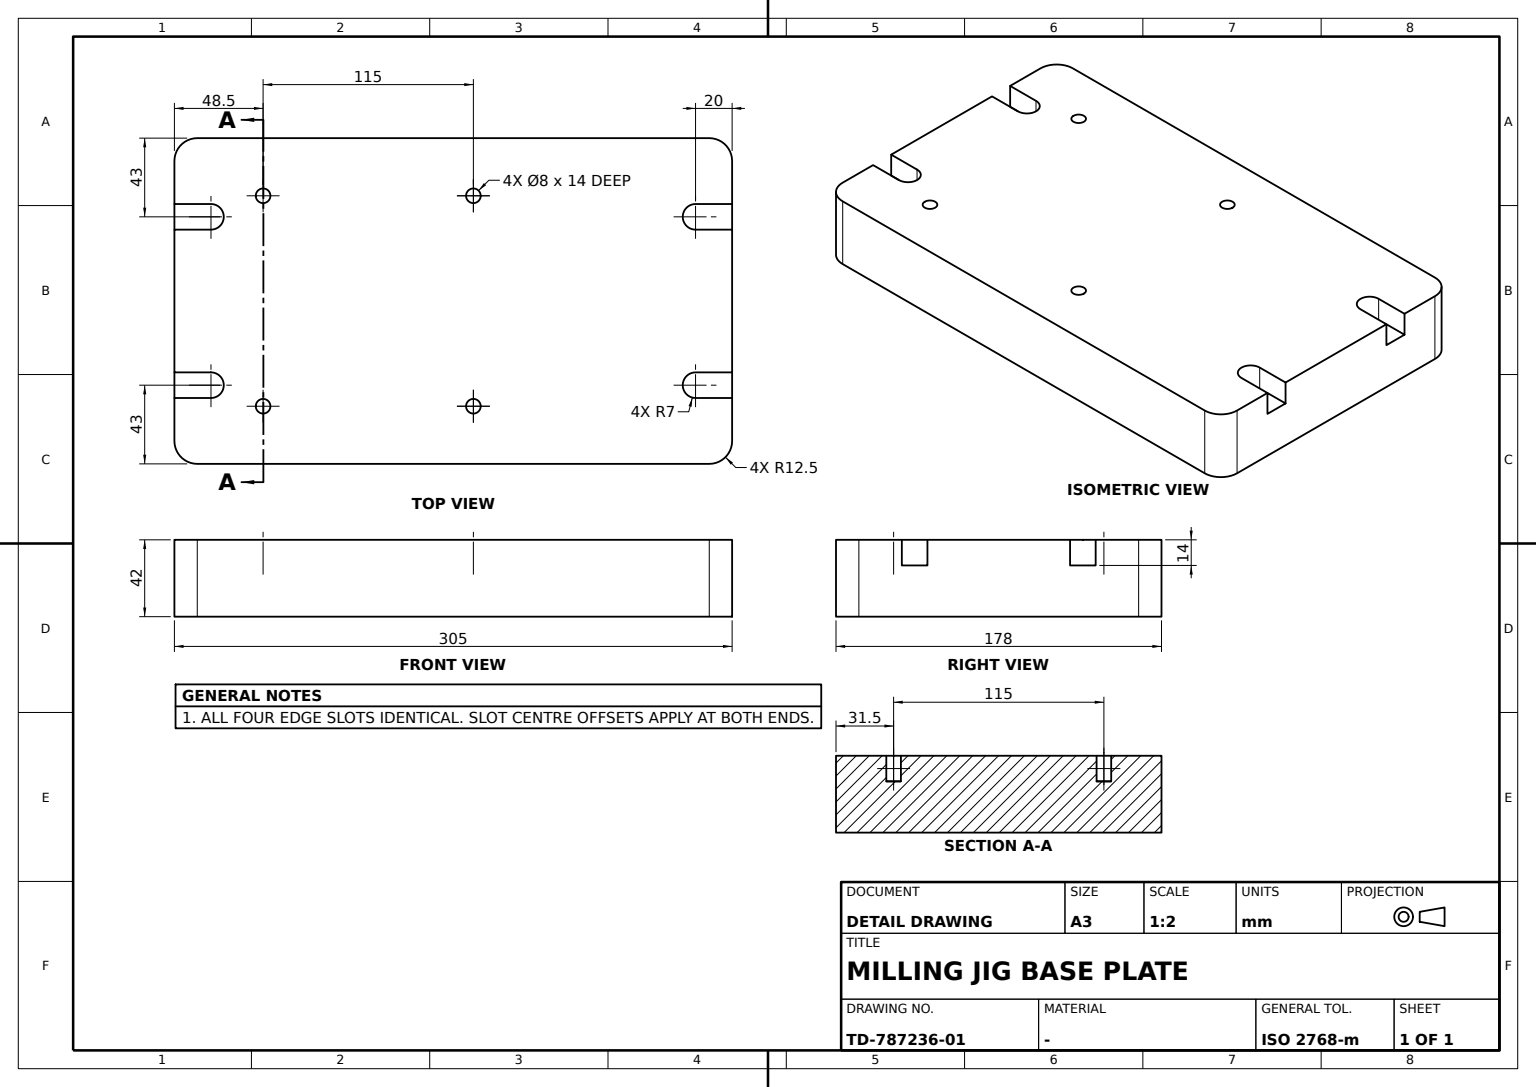
ISO-10303-21;
HEADER;
FILE_DESCRIPTION((''),'2;1');
FILE_NAME('','',(''),(''),'','','');
FILE_SCHEMA(('AUTOMOTIVE_DESIGN'));
ENDSEC;
DATA;
#1=APPLICATION_CONTEXT('');
#2=PRODUCT_CONTEXT('',#1,'mechanical');
#3=PRODUCT('','','',(#2));
#4=PRODUCT_DEFINITION_FORMATION('','',#3);
#5=PRODUCT_DEFINITION_CONTEXT('',#1,'design');
#6=PRODUCT_DEFINITION('','',#4,#5);
#7=PRODUCT_DEFINITION_SHAPE('','',#6);
#8=(LENGTH_UNIT()NAMED_UNIT(*)SI_UNIT(.MILLI.,.METRE.));
#9=(NAMED_UNIT(*)PLANE_ANGLE_UNIT()SI_UNIT($,.RADIAN.));
#10=(NAMED_UNIT(*)SI_UNIT($,.STERADIAN.)SOLID_ANGLE_UNIT());
#11=UNCERTAINTY_MEASURE_WITH_UNIT(LENGTH_MEASURE(1.E-05),#8,'distance_accuracy_value','');
#12=(GEOMETRIC_REPRESENTATION_CONTEXT(3)GLOBAL_UNCERTAINTY_ASSIGNED_CONTEXT((#11))GLOBAL_UNIT_ASSIGNED_CONTEXT((#8,#9,#10))REPRESENTATION_CONTEXT('',''));
#13=CARTESIAN_POINT('',(89.,140.,28.));
#14=VERTEX_POINT('',#13);
#15=CARTESIAN_POINT('',(89.,140.,-14.));
#16=VERTEX_POINT('',#15);
#17=CARTESIAN_POINT('',(89.,140.,7.));
#18=DIRECTION('',(0.,0.,-1.));
#19=VECTOR('',#18,1000.);
#20=LINE('',#17,#19);
#21=EDGE_CURVE('',#14,#16,#20,.T.);
#22=ORIENTED_EDGE('',*,*,#21,.F.);
#23=CARTESIAN_POINT('',(89.,-140.,28.));
#24=VERTEX_POINT('',#23);
#25=CARTESIAN_POINT('',(89.,0.,28.));
#26=DIRECTION('',(0.,1.,0.));
#27=VECTOR('',#26,1000.);
#28=LINE('',#25,#27);
#29=EDGE_CURVE('',#24,#14,#28,.T.);
#30=ORIENTED_EDGE('',*,*,#29,.F.);
#31=CARTESIAN_POINT('',(89.,-140.,-14.));
#32=VERTEX_POINT('',#31);
#33=CARTESIAN_POINT('',(89.,-140.,7.));
#34=LINE('',#33,#19);
#35=EDGE_CURVE('',#24,#32,#34,.T.);
#36=ORIENTED_EDGE('',*,*,#35,.T.);
#37=CARTESIAN_POINT('',(89.,0.,-14.));
#38=LINE('',#37,#27);
#39=EDGE_CURVE('',#32,#16,#38,.T.);
#40=ORIENTED_EDGE('',*,*,#39,.T.);
#41=EDGE_LOOP('',(#22,#30,#36,#40));
#42=FACE_OUTER_BOUND('',#41,.T.);
#43=CARTESIAN_POINT('',(89.,140.,0.));
#44=DIRECTION('',(1.,0.,0.));
#45=DIRECTION('',(0.,-1.,0.));
#46=AXIS2_PLACEMENT_3D('',#43,#44,#45);
#47=PLANE('',#46);
#48=ADVANCED_FACE('',(#42),#47,.T.);
#49=CARTESIAN_POINT('',(-89.,-140.,28.));
#50=VERTEX_POINT('',#49);
#51=CARTESIAN_POINT('',(-89.,-140.,-14.));
#52=VERTEX_POINT('',#51);
#53=CARTESIAN_POINT('',(-89.,-140.,7.));
#54=LINE('',#53,#19);
#55=EDGE_CURVE('',#50,#52,#54,.T.);
#56=ORIENTED_EDGE('',*,*,#55,.T.);
#57=CARTESIAN_POINT('',(-76.5,-152.5,-14.));
#58=VERTEX_POINT('',#57);
#59=CARTESIAN_POINT('',(-76.5,-140.,-14.));
#60=DIRECTION('',(0.,0.,1.));
#61=AXIS2_PLACEMENT_3D('',#59,#60,#26);
#62=CIRCLE('',#61,12.5);
#63=EDGE_CURVE('',#52,#58,#62,.T.);
#64=ORIENTED_EDGE('',*,*,#63,.T.);
#65=CARTESIAN_POINT('',(-76.5,-152.5,28.));
#66=VERTEX_POINT('',#65);
#67=CARTESIAN_POINT('',(-76.5,-152.5,7.));
#68=LINE('',#67,#19);
#69=EDGE_CURVE('',#66,#58,#68,.T.);
#70=ORIENTED_EDGE('',*,*,#69,.F.);
#71=CARTESIAN_POINT('',(-76.5,-140.,28.));
#72=AXIS2_PLACEMENT_3D('',#71,#60,#26);
#73=CIRCLE('',#72,12.5);
#74=EDGE_CURVE('',#50,#66,#73,.T.);
#75=ORIENTED_EDGE('',*,*,#74,.F.);
#76=EDGE_LOOP('',(#56,#64,#70,#75));
#77=FACE_OUTER_BOUND('',#76,.T.);
#78=CARTESIAN_POINT('',(-76.5,-140.,0.));
#79=AXIS2_PLACEMENT_3D('',#78,#18,#26);
#80=CYLINDRICAL_SURFACE('',#79,12.5);
#81=ADVANCED_FACE('',(#77),#80,.T.);
#82=CARTESIAN_POINT('',(-53.,132.5,0.));
#83=VERTEX_POINT('',#82);
#84=CARTESIAN_POINT('',(-53.,132.5,-14.));
#85=VERTEX_POINT('',#84);
#86=CARTESIAN_POINT('',(-53.,132.5,15.5));
#87=LINE('',#86,#19);
#88=EDGE_CURVE('',#83,#85,#87,.T.);
#89=ORIENTED_EDGE('',*,*,#88,.T.);
#90=CARTESIAN_POINT('',(-53.,152.5,-14.));
#91=VERTEX_POINT('',#90);
#92=CARTESIAN_POINT('',(-53.,142.5,-14.));
#93=VECTOR('',#45,1000.);
#94=LINE('',#92,#93);
#95=EDGE_CURVE('',#91,#85,#94,.T.);
#96=ORIENTED_EDGE('',*,*,#95,.F.);
#97=CARTESIAN_POINT('',(-53.,152.5,0.));
#98=VERTEX_POINT('',#97);
#99=CARTESIAN_POINT('',(-53.,152.5,-7.));
#100=LINE('',#99,#19);
#101=EDGE_CURVE('',#98,#91,#100,.T.);
#102=ORIENTED_EDGE('',*,*,#101,.F.);
#103=CARTESIAN_POINT('',(-53.,142.5,0.));
#104=LINE('',#103,#93);
#105=EDGE_CURVE('',#98,#83,#104,.T.);
#106=ORIENTED_EDGE('',*,*,#105,.T.);
#107=EDGE_LOOP('',(#89,#96,#102,#106));
#108=FACE_OUTER_BOUND('',#107,.T.);
#109=CARTESIAN_POINT('',(-53.,-132.5,14.));
#110=AXIS2_PLACEMENT_3D('',#109,#44,#45);
#111=PLANE('',#110);
#112=ADVANCED_FACE('',(#108),#111,.T.);
#113=CARTESIAN_POINT('',(76.5,-152.5,28.));
#114=VERTEX_POINT('',#113);
#115=CARTESIAN_POINT('',(0.,-152.5,28.));
#116=VECTOR('',#44,1000.);
#117=LINE('',#115,#116);
#118=EDGE_CURVE('',#66,#114,#117,.T.);
#119=ORIENTED_EDGE('',*,*,#118,.T.);
#120=CARTESIAN_POINT('',(76.5,-140.,28.));
#121=AXIS2_PLACEMENT_3D('',#120,#60,#26);
#122=CIRCLE('',#121,12.5);
#123=EDGE_CURVE('',#114,#24,#122,.T.);
#124=ORIENTED_EDGE('',*,*,#123,.T.);
#125=ORIENTED_EDGE('',*,*,#29,.T.);
#126=CARTESIAN_POINT('',(76.5,152.5,28.));
#127=VERTEX_POINT('',#126);
#128=CARTESIAN_POINT('',(76.5,140.,28.));
#129=AXIS2_PLACEMENT_3D('',#128,#60,#26);
#130=CIRCLE('',#129,12.5);
#131=EDGE_CURVE('',#14,#127,#130,.T.);
#132=ORIENTED_EDGE('',*,*,#131,.T.);
#133=CARTESIAN_POINT('',(-76.5,152.5,28.));
#134=VERTEX_POINT('',#133);
#135=CARTESIAN_POINT('',(0.,152.5,28.));
#136=DIRECTION('',(-1.,0.,0.));
#137=VECTOR('',#136,1000.);
#138=LINE('',#135,#137);
#139=EDGE_CURVE('',#127,#134,#138,.T.);
#140=ORIENTED_EDGE('',*,*,#139,.T.);
#141=CARTESIAN_POINT('',(-89.,140.,28.));
#142=VERTEX_POINT('',#141);
#143=CARTESIAN_POINT('',(-76.5,140.,28.));
#144=AXIS2_PLACEMENT_3D('',#143,#60,#26);
#145=CIRCLE('',#144,12.5);
#146=EDGE_CURVE('',#134,#142,#145,.T.);
#147=ORIENTED_EDGE('',*,*,#146,.T.);
#148=CARTESIAN_POINT('',(-89.,0.,28.));
#149=LINE('',#148,#93);
#150=EDGE_CURVE('',#142,#50,#149,.T.);
#151=ORIENTED_EDGE('',*,*,#150,.T.);
#152=ORIENTED_EDGE('',*,*,#74,.T.);
#153=EDGE_LOOP('',(#119,#124,#125,#132,#140,#147,#151,#152));
#154=FACE_OUTER_BOUND('',#153,.T.);
#155=CARTESIAN_POINT('',(0.,0.,28.));
#156=AXIS2_PLACEMENT_3D('',#155,#60,#26);
#157=PLANE('',#156);
#158=ADVANCED_FACE('',(#154),#157,.T.);
#159=CARTESIAN_POINT('',(-57.5,-108.,0.));
#160=VERTEX_POINT('',#159);
#161=CARTESIAN_POINT('',(-57.5,-100.,0.));
#162=VERTEX_POINT('',#161);
#163=CARTESIAN_POINT('',(-57.5,-104.,0.));
#164=AXIS2_PLACEMENT_3D('',#163,#60,#26);
#165=CIRCLE('',#164,4.);
#166=EDGE_CURVE('',#160,#162,#165,.T.);
#167=ORIENTED_EDGE('',*,*,#166,.T.);
#168=CARTESIAN_POINT('',(-57.5,-100.,-14.));
#169=VERTEX_POINT('',#168);
#170=CARTESIAN_POINT('',(-57.5,-100.,0.84));
#171=LINE('',#170,#19);
#172=EDGE_CURVE('',#162,#169,#171,.T.);
#173=ORIENTED_EDGE('',*,*,#172,.T.);
#174=CARTESIAN_POINT('',(-57.5,-108.,-14.));
#175=VERTEX_POINT('',#174);
#176=CARTESIAN_POINT('',(-57.5,-104.,-14.));
#177=AXIS2_PLACEMENT_3D('',#176,#60,#26);
#178=CIRCLE('',#177,4.);
#179=EDGE_CURVE('',#175,#169,#178,.T.);
#180=ORIENTED_EDGE('',*,*,#179,.F.);
#181=CARTESIAN_POINT('',(-57.5,-108.,0.84));
#182=LINE('',#181,#19);
#183=EDGE_CURVE('',#160,#175,#182,.T.);
#184=ORIENTED_EDGE('',*,*,#183,.F.);
#185=EDGE_LOOP('',(#167,#173,#180,#184));
#186=FACE_OUTER_BOUND('',#185,.T.);
#187=CARTESIAN_POINT('',(-57.5,-104.,0.84));
#188=AXIS2_PLACEMENT_3D('',#187,#18,#26);
#189=CYLINDRICAL_SURFACE('',#188,4.);
#190=ADVANCED_FACE('',(#186),#189,.F.);
#191=CARTESIAN_POINT('',(-39.,132.5,0.));
#192=VERTEX_POINT('',#191);
#193=CARTESIAN_POINT('',(-46.,132.5,0.));
#194=AXIS2_PLACEMENT_3D('',#193,#60,#26);
#195=CIRCLE('',#194,7.);
#196=EDGE_CURVE('',#83,#192,#195,.T.);
#197=ORIENTED_EDGE('',*,*,#196,.T.);
#198=CARTESIAN_POINT('',(-39.,132.5,-14.));
#199=VERTEX_POINT('',#198);
#200=CARTESIAN_POINT('',(-39.,132.5,15.5));
#201=LINE('',#200,#19);
#202=EDGE_CURVE('',#192,#199,#201,.T.);
#203=ORIENTED_EDGE('',*,*,#202,.T.);
#204=CARTESIAN_POINT('',(-46.,132.5,-14.));
#205=AXIS2_PLACEMENT_3D('',#204,#60,#26);
#206=CIRCLE('',#205,7.);
#207=EDGE_CURVE('',#85,#199,#206,.T.);
#208=ORIENTED_EDGE('',*,*,#207,.F.);
#209=ORIENTED_EDGE('',*,*,#88,.F.);
#210=EDGE_LOOP('',(#197,#203,#208,#209));
#211=FACE_OUTER_BOUND('',#210,.T.);
#212=CARTESIAN_POINT('',(-46.,132.5,15.5));
#213=AXIS2_PLACEMENT_3D('',#212,#18,#26);
#214=CYLINDRICAL_SURFACE('',#213,7.);
#215=ADVANCED_FACE('',(#211),#214,.F.);
#216=CARTESIAN_POINT('',(-57.5,15.,0.));
#217=VERTEX_POINT('',#216);
#218=CARTESIAN_POINT('',(-57.5,15.,-14.));
#219=VERTEX_POINT('',#218);
#220=CARTESIAN_POINT('',(-57.5,15.,0.84));
#221=LINE('',#220,#19);
#222=EDGE_CURVE('',#217,#219,#221,.T.);
#223=ORIENTED_EDGE('',*,*,#222,.F.);
#224=CARTESIAN_POINT('',(-57.5,7.,0.));
#225=VERTEX_POINT('',#224);
#226=CARTESIAN_POINT('',(-57.5,11.,0.));
#227=AXIS2_PLACEMENT_3D('',#226,#60,#26);
#228=CIRCLE('',#227,4.);
#229=EDGE_CURVE('',#217,#225,#228,.T.);
#230=ORIENTED_EDGE('',*,*,#229,.T.);
#231=CARTESIAN_POINT('',(-57.5,7.,-14.));
#232=VERTEX_POINT('',#231);
#233=CARTESIAN_POINT('',(-57.5,7.,0.84));
#234=LINE('',#233,#19);
#235=EDGE_CURVE('',#225,#232,#234,.T.);
#236=ORIENTED_EDGE('',*,*,#235,.T.);
#237=CARTESIAN_POINT('',(-57.5,11.,-14.));
#238=AXIS2_PLACEMENT_3D('',#237,#60,#26);
#239=CIRCLE('',#238,4.);
#240=EDGE_CURVE('',#219,#232,#239,.T.);
#241=ORIENTED_EDGE('',*,*,#240,.F.);
#242=EDGE_LOOP('',(#223,#230,#236,#241));
#243=FACE_OUTER_BOUND('',#242,.T.);
#244=CARTESIAN_POINT('',(-57.5,11.,0.84));
#245=AXIS2_PLACEMENT_3D('',#244,#18,#26);
#246=CYLINDRICAL_SURFACE('',#245,4.);
#247=ADVANCED_FACE('',(#243),#246,.F.);
#248=CARTESIAN_POINT('',(76.5,152.5,-14.));
#249=VERTEX_POINT('',#248);
#250=CARTESIAN_POINT('',(76.5,152.5,7.));
#251=LINE('',#250,#19);
#252=EDGE_CURVE('',#127,#249,#251,.T.);
#253=ORIENTED_EDGE('',*,*,#252,.T.);
#254=CARTESIAN_POINT('',(53.,152.5,-14.));
#255=VERTEX_POINT('',#254);
#256=CARTESIAN_POINT('',(64.75,152.5,-14.));
#257=LINE('',#256,#137);
#258=EDGE_CURVE('',#249,#255,#257,.T.);
#259=ORIENTED_EDGE('',*,*,#258,.T.);
#260=CARTESIAN_POINT('',(53.,152.5,0.));
#261=VERTEX_POINT('',#260);
#262=CARTESIAN_POINT('',(53.,152.5,-7.));
#263=LINE('',#262,#19);
#264=EDGE_CURVE('',#261,#255,#263,.T.);
#265=ORIENTED_EDGE('',*,*,#264,.F.);
#266=CARTESIAN_POINT('',(39.,152.5,0.));
#267=VERTEX_POINT('',#266);
#268=CARTESIAN_POINT('',(46.,152.5,0.));
#269=LINE('',#268,#137);
#270=EDGE_CURVE('',#261,#267,#269,.T.);
#271=ORIENTED_EDGE('',*,*,#270,.T.);
#272=CARTESIAN_POINT('',(39.,152.5,-14.));
#273=VERTEX_POINT('',#272);
#274=CARTESIAN_POINT('',(39.,152.5,-7.));
#275=LINE('',#274,#19);
#276=EDGE_CURVE('',#267,#273,#275,.T.);
#277=ORIENTED_EDGE('',*,*,#276,.T.);
#278=CARTESIAN_POINT('',(-39.,152.5,-14.));
#279=VERTEX_POINT('',#278);
#280=CARTESIAN_POINT('',(0.,152.5,-14.));
#281=LINE('',#280,#137);
#282=EDGE_CURVE('',#273,#279,#281,.T.);
#283=ORIENTED_EDGE('',*,*,#282,.T.);
#284=CARTESIAN_POINT('',(-39.,152.5,0.));
#285=VERTEX_POINT('',#284);
#286=CARTESIAN_POINT('',(-39.,152.5,-7.));
#287=LINE('',#286,#19);
#288=EDGE_CURVE('',#285,#279,#287,.T.);
#289=ORIENTED_EDGE('',*,*,#288,.F.);
#290=CARTESIAN_POINT('',(-46.,152.5,0.));
#291=LINE('',#290,#137);
#292=EDGE_CURVE('',#285,#98,#291,.T.);
#293=ORIENTED_EDGE('',*,*,#292,.T.);
#294=ORIENTED_EDGE('',*,*,#101,.T.);
#295=CARTESIAN_POINT('',(-76.5,152.5,-14.));
#296=VERTEX_POINT('',#295);
#297=CARTESIAN_POINT('',(-64.75,152.5,-14.));
#298=LINE('',#297,#137);
#299=EDGE_CURVE('',#91,#296,#298,.T.);
#300=ORIENTED_EDGE('',*,*,#299,.T.);
#301=CARTESIAN_POINT('',(-76.5,152.5,7.));
#302=LINE('',#301,#19);
#303=EDGE_CURVE('',#134,#296,#302,.T.);
#304=ORIENTED_EDGE('',*,*,#303,.F.);
#305=ORIENTED_EDGE('',*,*,#139,.F.);
#306=EDGE_LOOP('',(#253,#259,#265,#271,#277,#283,#289,#293,#294,#300,#304,#305));
#307=FACE_OUTER_BOUND('',#306,.T.);
#308=CARTESIAN_POINT('',(-76.5,152.5,0.));
#309=AXIS2_PLACEMENT_3D('',#308,#26,#44);
#310=PLANE('',#309);
#311=ADVANCED_FACE('',(#307),#310,.T.);
#312=ORIENTED_EDGE('',*,*,#202,.F.);
#313=CARTESIAN_POINT('',(-39.,142.5,0.));
#314=LINE('',#313,#93);
#315=EDGE_CURVE('',#285,#192,#314,.T.);
#316=ORIENTED_EDGE('',*,*,#315,.F.);
#317=ORIENTED_EDGE('',*,*,#288,.T.);
#318=CARTESIAN_POINT('',(-39.,142.5,-14.));
#319=LINE('',#318,#93);
#320=EDGE_CURVE('',#279,#199,#319,.T.);
#321=ORIENTED_EDGE('',*,*,#320,.T.);
#322=EDGE_LOOP('',(#312,#316,#317,#321));
#323=FACE_OUTER_BOUND('',#322,.T.);
#324=CARTESIAN_POINT('',(-39.,-132.5,14.));
#325=AXIS2_PLACEMENT_3D('',#324,#44,#45);
#326=PLANE('',#325);
#327=ADVANCED_FACE('',(#323),#326,.F.);
#328=EDGE_CURVE('',#225,#217,#228,.T.);
#329=ORIENTED_EDGE('',*,*,#328,.T.);
#330=ORIENTED_EDGE('',*,*,#222,.T.);
#331=EDGE_CURVE('',#232,#219,#239,.T.);
#332=ORIENTED_EDGE('',*,*,#331,.F.);
#333=ORIENTED_EDGE('',*,*,#235,.F.);
#334=EDGE_LOOP('',(#329,#330,#332,#333));
#335=FACE_OUTER_BOUND('',#334,.T.);
#336=ADVANCED_FACE('',(#335),#246,.F.);
#337=CARTESIAN_POINT('',(53.,132.5,0.));
#338=VERTEX_POINT('',#337);
#339=CARTESIAN_POINT('',(53.,142.5,0.));
#340=LINE('',#339,#93);
#341=EDGE_CURVE('',#261,#338,#340,.T.);
#342=ORIENTED_EDGE('',*,*,#341,.T.);
#343=CARTESIAN_POINT('',(46.,125.5,0.));
#344=VERTEX_POINT('',#343);
#345=CARTESIAN_POINT('',(46.,132.5,0.));
#346=AXIS2_PLACEMENT_3D('',#345,#60,#26);
#347=CIRCLE('',#346,7.);
#348=EDGE_CURVE('',#344,#338,#347,.T.);
#349=ORIENTED_EDGE('',*,*,#348,.F.);
#350=CARTESIAN_POINT('',(39.,132.5,0.));
#351=VERTEX_POINT('',#350);
#352=EDGE_CURVE('',#351,#344,#347,.T.);
#353=ORIENTED_EDGE('',*,*,#352,.F.);
#354=CARTESIAN_POINT('',(39.,142.5,0.));
#355=LINE('',#354,#93);
#356=EDGE_CURVE('',#267,#351,#355,.T.);
#357=ORIENTED_EDGE('',*,*,#356,.F.);
#358=ORIENTED_EDGE('',*,*,#270,.F.);
#359=EDGE_LOOP('',(#342,#349,#353,#357,#358));
#360=FACE_OUTER_BOUND('',#359,.T.);
#361=CARTESIAN_POINT('',(0.,0.,0.));
#362=AXIS2_PLACEMENT_3D('',#361,#60,#26);
#363=PLANE('',#362);
#364=ADVANCED_FACE('',(#360),#363,.F.);
#365=CARTESIAN_POINT('',(39.,132.5,-14.));
#366=VERTEX_POINT('',#365);
#367=CARTESIAN_POINT('',(39.,132.5,-7.));
#368=LINE('',#367,#19);
#369=EDGE_CURVE('',#351,#366,#368,.T.);
#370=ORIENTED_EDGE('',*,*,#369,.T.);
#371=CARTESIAN_POINT('',(39.,142.5,-14.));
#372=LINE('',#371,#93);
#373=EDGE_CURVE('',#273,#366,#372,.T.);
#374=ORIENTED_EDGE('',*,*,#373,.F.);
#375=ORIENTED_EDGE('',*,*,#276,.F.);
#376=ORIENTED_EDGE('',*,*,#356,.T.);
#377=EDGE_LOOP('',(#370,#374,#375,#376));
#378=FACE_OUTER_BOUND('',#377,.T.);
#379=CARTESIAN_POINT('',(39.,-132.5,14.));
#380=AXIS2_PLACEMENT_3D('',#379,#44,#45);
#381=PLANE('',#380);
#382=ADVANCED_FACE('',(#378),#381,.T.);
#383=CARTESIAN_POINT('',(-39.,-132.5,-14.));
#384=VERTEX_POINT('',#383);
#385=CARTESIAN_POINT('',(-46.,-125.5,-14.));
#386=VERTEX_POINT('',#385);
#387=CARTESIAN_POINT('',(-46.,-132.5,-14.));
#388=AXIS2_PLACEMENT_3D('',#387,#60,#26);
#389=CIRCLE('',#388,7.);
#390=EDGE_CURVE('',#384,#386,#389,.T.);
#391=ORIENTED_EDGE('',*,*,#390,.F.);
#392=CARTESIAN_POINT('',(-39.,-132.5,0.));
#393=VERTEX_POINT('',#392);
#394=CARTESIAN_POINT('',(-39.,-132.5,0.84));
#395=LINE('',#394,#19);
#396=EDGE_CURVE('',#393,#384,#395,.T.);
#397=ORIENTED_EDGE('',*,*,#396,.F.);
#398=CARTESIAN_POINT('',(-46.,-125.5,0.));
#399=VERTEX_POINT('',#398);
#400=CARTESIAN_POINT('',(-46.,-132.5,0.));
#401=AXIS2_PLACEMENT_3D('',#400,#60,#26);
#402=CIRCLE('',#401,7.);
#403=EDGE_CURVE('',#393,#399,#402,.T.);
#404=ORIENTED_EDGE('',*,*,#403,.T.);
#405=CARTESIAN_POINT('',(-46.,-125.5,-0.66));
#406=LINE('',#405,#19);
#407=EDGE_CURVE('',#399,#386,#406,.T.);
#408=ORIENTED_EDGE('',*,*,#407,.T.);
#409=EDGE_LOOP('',(#391,#397,#404,#408));
#410=FACE_OUTER_BOUND('',#409,.T.);
#411=CARTESIAN_POINT('',(-46.,-132.5,-0.66));
#412=AXIS2_PLACEMENT_3D('',#411,#18,#26);
#413=CYLINDRICAL_SURFACE('',#412,7.);
#414=ADVANCED_FACE('',(#410),#413,.F.);
#415=ORIENTED_EDGE('',*,*,#403,.F.);
#416=CARTESIAN_POINT('',(-39.,-152.5,0.));
#417=VERTEX_POINT('',#416);
#418=CARTESIAN_POINT('',(-39.,-142.5,0.));
#419=LINE('',#418,#27);
#420=EDGE_CURVE('',#417,#393,#419,.T.);
#421=ORIENTED_EDGE('',*,*,#420,.F.);
#422=CARTESIAN_POINT('',(-53.,-152.5,0.));
#423=VERTEX_POINT('',#422);
#424=CARTESIAN_POINT('',(-46.,-152.5,0.));
#425=LINE('',#424,#116);
#426=EDGE_CURVE('',#423,#417,#425,.T.);
#427=ORIENTED_EDGE('',*,*,#426,.F.);
#428=CARTESIAN_POINT('',(-53.,-132.5,0.));
#429=VERTEX_POINT('',#428);
#430=CARTESIAN_POINT('',(-53.,-142.5,0.));
#431=LINE('',#430,#27);
#432=EDGE_CURVE('',#423,#429,#431,.T.);
#433=ORIENTED_EDGE('',*,*,#432,.T.);
#434=EDGE_CURVE('',#399,#429,#402,.T.);
#435=ORIENTED_EDGE('',*,*,#434,.F.);
#436=EDGE_LOOP('',(#415,#421,#427,#433,#435));
#437=FACE_OUTER_BOUND('',#436,.T.);
#438=ADVANCED_FACE('',(#437),#363,.F.);
#439=CARTESIAN_POINT('',(57.5,7.,0.));
#440=VERTEX_POINT('',#439);
#441=CARTESIAN_POINT('',(57.5,7.,-14.));
#442=VERTEX_POINT('',#441);
#443=CARTESIAN_POINT('',(57.5,7.,0.84));
#444=LINE('',#443,#19);
#445=EDGE_CURVE('',#440,#442,#444,.T.);
#446=ORIENTED_EDGE('',*,*,#445,.T.);
#447=CARTESIAN_POINT('',(57.5,15.,-14.));
#448=VERTEX_POINT('',#447);
#449=CARTESIAN_POINT('',(57.5,11.,-14.));
#450=AXIS2_PLACEMENT_3D('',#449,#60,#26);
#451=CIRCLE('',#450,4.);
#452=EDGE_CURVE('',#448,#442,#451,.T.);
#453=ORIENTED_EDGE('',*,*,#452,.F.);
#454=CARTESIAN_POINT('',(57.5,15.,0.));
#455=VERTEX_POINT('',#454);
#456=CARTESIAN_POINT('',(57.5,15.,0.84));
#457=LINE('',#456,#19);
#458=EDGE_CURVE('',#455,#448,#457,.T.);
#459=ORIENTED_EDGE('',*,*,#458,.F.);
#460=CARTESIAN_POINT('',(57.5,11.,0.));
#461=AXIS2_PLACEMENT_3D('',#460,#60,#26);
#462=CIRCLE('',#461,4.);
#463=EDGE_CURVE('',#455,#440,#462,.T.);
#464=ORIENTED_EDGE('',*,*,#463,.T.);
#465=EDGE_LOOP('',(#446,#453,#459,#464));
#466=FACE_OUTER_BOUND('',#465,.T.);
#467=CARTESIAN_POINT('',(57.5,11.,0.84));
#468=AXIS2_PLACEMENT_3D('',#467,#18,#26);
#469=CYLINDRICAL_SURFACE('',#468,4.);
#470=ADVANCED_FACE('',(#466),#469,.F.);
#471=CARTESIAN_POINT('',(46.,125.5,-14.));
#472=VERTEX_POINT('',#471);
#473=CARTESIAN_POINT('',(46.,125.5,-0.66));
#474=VECTOR('',#60,1000.);
#475=LINE('',#473,#474);
#476=EDGE_CURVE('',#472,#344,#475,.T.);
#477=ORIENTED_EDGE('',*,*,#476,.F.);
#478=CARTESIAN_POINT('',(46.,132.5,-14.));
#479=AXIS2_PLACEMENT_3D('',#478,#60,#26);
#480=CIRCLE('',#479,7.);
#481=EDGE_CURVE('',#366,#472,#480,.T.);
#482=ORIENTED_EDGE('',*,*,#481,.F.);
#483=ORIENTED_EDGE('',*,*,#369,.F.);
#484=ORIENTED_EDGE('',*,*,#352,.T.);
#485=EDGE_LOOP('',(#477,#482,#483,#484));
#486=FACE_OUTER_BOUND('',#485,.T.);
#487=CARTESIAN_POINT('',(46.,132.5,-0.66));
#488=AXIS2_PLACEMENT_3D('',#487,#60,#45);
#489=CYLINDRICAL_SURFACE('',#488,7.);
#490=ADVANCED_FACE('',(#486),#489,.F.);
#491=CARTESIAN_POINT('',(-53.,-152.5,-14.));
#492=VERTEX_POINT('',#491);
#493=CARTESIAN_POINT('',(-64.75,-152.5,-14.));
#494=LINE('',#493,#116);
#495=EDGE_CURVE('',#58,#492,#494,.T.);
#496=ORIENTED_EDGE('',*,*,#495,.T.);
#497=CARTESIAN_POINT('',(-53.,-152.5,-7.));
#498=LINE('',#497,#19);
#499=EDGE_CURVE('',#423,#492,#498,.T.);
#500=ORIENTED_EDGE('',*,*,#499,.F.);
#501=ORIENTED_EDGE('',*,*,#426,.T.);
#502=CARTESIAN_POINT('',(-39.,-152.5,-14.));
#503=VERTEX_POINT('',#502);
#504=CARTESIAN_POINT('',(-39.,-152.5,-7.));
#505=LINE('',#504,#19);
#506=EDGE_CURVE('',#417,#503,#505,.T.);
#507=ORIENTED_EDGE('',*,*,#506,.T.);
#508=CARTESIAN_POINT('',(39.,-152.5,-14.));
#509=VERTEX_POINT('',#508);
#510=CARTESIAN_POINT('',(0.,-152.5,-14.));
#511=LINE('',#510,#116);
#512=EDGE_CURVE('',#503,#509,#511,.T.);
#513=ORIENTED_EDGE('',*,*,#512,.T.);
#514=CARTESIAN_POINT('',(39.,-152.5,0.));
#515=VERTEX_POINT('',#514);
#516=CARTESIAN_POINT('',(39.,-152.5,-7.));
#517=LINE('',#516,#19);
#518=EDGE_CURVE('',#515,#509,#517,.T.);
#519=ORIENTED_EDGE('',*,*,#518,.F.);
#520=CARTESIAN_POINT('',(53.,-152.5,0.));
#521=VERTEX_POINT('',#520);
#522=CARTESIAN_POINT('',(46.,-152.5,0.));
#523=LINE('',#522,#116);
#524=EDGE_CURVE('',#515,#521,#523,.T.);
#525=ORIENTED_EDGE('',*,*,#524,.T.);
#526=CARTESIAN_POINT('',(53.,-152.5,-14.));
#527=VERTEX_POINT('',#526);
#528=CARTESIAN_POINT('',(53.,-152.5,-7.));
#529=LINE('',#528,#19);
#530=EDGE_CURVE('',#521,#527,#529,.T.);
#531=ORIENTED_EDGE('',*,*,#530,.T.);
#532=CARTESIAN_POINT('',(76.5,-152.5,-14.));
#533=VERTEX_POINT('',#532);
#534=CARTESIAN_POINT('',(64.75,-152.5,-14.));
#535=LINE('',#534,#116);
#536=EDGE_CURVE('',#527,#533,#535,.T.);
#537=ORIENTED_EDGE('',*,*,#536,.T.);
#538=CARTESIAN_POINT('',(76.5,-152.5,7.));
#539=LINE('',#538,#19);
#540=EDGE_CURVE('',#114,#533,#539,.T.);
#541=ORIENTED_EDGE('',*,*,#540,.F.);
#542=ORIENTED_EDGE('',*,*,#118,.F.);
#543=ORIENTED_EDGE('',*,*,#69,.T.);
#544=EDGE_LOOP('',(#496,#500,#501,#507,#513,#519,#525,#531,#537,#541,#542,#543));
#545=FACE_OUTER_BOUND('',#544,.T.);
#546=CARTESIAN_POINT('',(76.5,-152.5,0.));
#547=AXIS2_PLACEMENT_3D('',#546,#45,#136);
#548=PLANE('',#547);
#549=ADVANCED_FACE('',(#545),#548,.T.);
#550=ORIENTED_EDGE('',*,*,#55,.F.);
#551=ORIENTED_EDGE('',*,*,#150,.F.);
#552=CARTESIAN_POINT('',(-89.,140.,-14.));
#553=VERTEX_POINT('',#552);
#554=CARTESIAN_POINT('',(-89.,140.,7.));
#555=LINE('',#554,#19);
#556=EDGE_CURVE('',#142,#553,#555,.T.);
#557=ORIENTED_EDGE('',*,*,#556,.T.);
#558=CARTESIAN_POINT('',(-89.,0.,-14.));
#559=LINE('',#558,#93);
#560=EDGE_CURVE('',#553,#52,#559,.T.);
#561=ORIENTED_EDGE('',*,*,#560,.T.);
#562=EDGE_LOOP('',(#550,#551,#557,#561));
#563=FACE_OUTER_BOUND('',#562,.T.);
#564=CARTESIAN_POINT('',(-89.,-140.,0.));
#565=AXIS2_PLACEMENT_3D('',#564,#136,#26);
#566=PLANE('',#565);
#567=ADVANCED_FACE('',(#563),#566,.T.);
#568=CARTESIAN_POINT('',(53.,132.5,-14.));
#569=VERTEX_POINT('',#568);
#570=CARTESIAN_POINT('',(53.,132.5,-7.));
#571=LINE('',#570,#19);
#572=EDGE_CURVE('',#338,#569,#571,.T.);
#573=ORIENTED_EDGE('',*,*,#572,.T.);
#574=EDGE_CURVE('',#472,#569,#480,.T.);
#575=ORIENTED_EDGE('',*,*,#574,.F.);
#576=ORIENTED_EDGE('',*,*,#476,.T.);
#577=ORIENTED_EDGE('',*,*,#348,.T.);
#578=EDGE_LOOP('',(#573,#575,#576,#577));
#579=FACE_OUTER_BOUND('',#578,.T.);
#580=ADVANCED_FACE('',(#579),#489,.F.);
#581=ORIENTED_EDGE('',*,*,#540,.T.);
#582=CARTESIAN_POINT('',(76.5,-140.,-14.));
#583=AXIS2_PLACEMENT_3D('',#582,#60,#26);
#584=CIRCLE('',#583,12.5);
#585=EDGE_CURVE('',#533,#32,#584,.T.);
#586=ORIENTED_EDGE('',*,*,#585,.T.);
#587=ORIENTED_EDGE('',*,*,#35,.F.);
#588=ORIENTED_EDGE('',*,*,#123,.F.);
#589=EDGE_LOOP('',(#581,#586,#587,#588));
#590=FACE_OUTER_BOUND('',#589,.T.);
#591=CARTESIAN_POINT('',(76.5,-140.,0.));
#592=AXIS2_PLACEMENT_3D('',#591,#18,#26);
#593=CYLINDRICAL_SURFACE('',#592,12.5);
#594=ADVANCED_FACE('',(#590),#593,.T.);
#595=ORIENTED_EDGE('',*,*,#445,.F.);
#596=EDGE_CURVE('',#440,#455,#462,.T.);
#597=ORIENTED_EDGE('',*,*,#596,.T.);
#598=ORIENTED_EDGE('',*,*,#458,.T.);
#599=EDGE_CURVE('',#442,#448,#451,.T.);
#600=ORIENTED_EDGE('',*,*,#599,.F.);
#601=EDGE_LOOP('',(#595,#597,#598,#600));
#602=FACE_OUTER_BOUND('',#601,.T.);
#603=ADVANCED_FACE('',(#602),#469,.F.);
#604=CARTESIAN_POINT('',(-53.,-132.5,-14.));
#605=VERTEX_POINT('',#604);
#606=EDGE_CURVE('',#386,#605,#389,.T.);
#607=ORIENTED_EDGE('',*,*,#606,.F.);
#608=ORIENTED_EDGE('',*,*,#407,.F.);
#609=ORIENTED_EDGE('',*,*,#434,.T.);
#610=CARTESIAN_POINT('',(-53.,-132.5,0.84));
#611=LINE('',#610,#19);
#612=EDGE_CURVE('',#429,#605,#611,.T.);
#613=ORIENTED_EDGE('',*,*,#612,.T.);
#614=EDGE_LOOP('',(#607,#608,#609,#613));
#615=FACE_OUTER_BOUND('',#614,.T.);
#616=ADVANCED_FACE('',(#615),#413,.F.);
#617=CARTESIAN_POINT('',(57.5,-100.,0.));
#618=VERTEX_POINT('',#617);
#619=CARTESIAN_POINT('',(57.5,-108.,0.));
#620=VERTEX_POINT('',#619);
#621=CARTESIAN_POINT('',(57.5,-104.,0.));
#622=AXIS2_PLACEMENT_3D('',#621,#60,#26);
#623=CIRCLE('',#622,4.);
#624=EDGE_CURVE('',#618,#620,#623,.T.);
#625=ORIENTED_EDGE('',*,*,#624,.T.);
#626=CARTESIAN_POINT('',(57.5,-108.,-14.));
#627=VERTEX_POINT('',#626);
#628=CARTESIAN_POINT('',(57.5,-108.,0.84));
#629=LINE('',#628,#19);
#630=EDGE_CURVE('',#620,#627,#629,.T.);
#631=ORIENTED_EDGE('',*,*,#630,.T.);
#632=CARTESIAN_POINT('',(57.5,-100.,-14.));
#633=VERTEX_POINT('',#632);
#634=CARTESIAN_POINT('',(57.5,-104.,-14.));
#635=AXIS2_PLACEMENT_3D('',#634,#60,#26);
#636=CIRCLE('',#635,4.);
#637=EDGE_CURVE('',#633,#627,#636,.T.);
#638=ORIENTED_EDGE('',*,*,#637,.F.);
#639=CARTESIAN_POINT('',(57.5,-100.,0.84));
#640=LINE('',#639,#19);
#641=EDGE_CURVE('',#618,#633,#640,.T.);
#642=ORIENTED_EDGE('',*,*,#641,.F.);
#643=EDGE_LOOP('',(#625,#631,#638,#642));
#644=FACE_OUTER_BOUND('',#643,.T.);
#645=CARTESIAN_POINT('',(57.5,-104.,0.84));
#646=AXIS2_PLACEMENT_3D('',#645,#18,#26);
#647=CYLINDRICAL_SURFACE('',#646,4.);
#648=ADVANCED_FACE('',(#644),#647,.F.);
#649=CARTESIAN_POINT('',(53.,142.5,-14.));
#650=LINE('',#649,#93);
#651=EDGE_CURVE('',#255,#569,#650,.T.);
#652=ORIENTED_EDGE('',*,*,#651,.T.);
#653=ORIENTED_EDGE('',*,*,#572,.F.);
#654=ORIENTED_EDGE('',*,*,#341,.F.);
#655=ORIENTED_EDGE('',*,*,#264,.T.);
#656=EDGE_LOOP('',(#652,#653,#654,#655));
#657=FACE_OUTER_BOUND('',#656,.T.);
#658=CARTESIAN_POINT('',(53.,-132.5,14.));
#659=AXIS2_PLACEMENT_3D('',#658,#44,#45);
#660=PLANE('',#659);
#661=ADVANCED_FACE('',(#657),#660,.F.);
#662=CARTESIAN_POINT('',(46.,-125.5,0.));
#663=VERTEX_POINT('',#662);
#664=CARTESIAN_POINT('',(39.,-132.5,0.));
#665=VERTEX_POINT('',#664);
#666=CARTESIAN_POINT('',(46.,-132.5,0.));
#667=AXIS2_PLACEMENT_3D('',#666,#60,#26);
#668=CIRCLE('',#667,7.);
#669=EDGE_CURVE('',#663,#665,#668,.T.);
#670=ORIENTED_EDGE('',*,*,#669,.T.);
#671=CARTESIAN_POINT('',(39.,-132.5,-14.));
#672=VERTEX_POINT('',#671);
#673=CARTESIAN_POINT('',(39.,-132.5,-7.));
#674=LINE('',#673,#19);
#675=EDGE_CURVE('',#665,#672,#674,.T.);
#676=ORIENTED_EDGE('',*,*,#675,.T.);
#677=CARTESIAN_POINT('',(46.,-125.5,-14.));
#678=VERTEX_POINT('',#677);
#679=CARTESIAN_POINT('',(46.,-132.5,-14.));
#680=AXIS2_PLACEMENT_3D('',#679,#60,#26);
#681=CIRCLE('',#680,7.);
#682=EDGE_CURVE('',#678,#672,#681,.T.);
#683=ORIENTED_EDGE('',*,*,#682,.F.);
#684=CARTESIAN_POINT('',(46.,-125.5,15.5));
#685=LINE('',#684,#474);
#686=EDGE_CURVE('',#678,#663,#685,.T.);
#687=ORIENTED_EDGE('',*,*,#686,.T.);
#688=EDGE_LOOP('',(#670,#676,#683,#687));
#689=FACE_OUTER_BOUND('',#688,.T.);
#690=CARTESIAN_POINT('',(46.,-132.5,15.5));
#691=AXIS2_PLACEMENT_3D('',#690,#60,#26);
#692=CYLINDRICAL_SURFACE('',#691,7.);
#693=ADVANCED_FACE('',(#689),#692,.F.);
#694=ORIENTED_EDGE('',*,*,#686,.F.);
#695=CARTESIAN_POINT('',(53.,-132.5,-14.));
#696=VERTEX_POINT('',#695);
#697=EDGE_CURVE('',#696,#678,#681,.T.);
#698=ORIENTED_EDGE('',*,*,#697,.F.);
#699=CARTESIAN_POINT('',(53.,-132.5,0.));
#700=VERTEX_POINT('',#699);
#701=CARTESIAN_POINT('',(53.,-132.5,-7.));
#702=LINE('',#701,#19);
#703=EDGE_CURVE('',#700,#696,#702,.T.);
#704=ORIENTED_EDGE('',*,*,#703,.F.);
#705=EDGE_CURVE('',#700,#663,#668,.T.);
#706=ORIENTED_EDGE('',*,*,#705,.T.);
#707=EDGE_LOOP('',(#694,#698,#704,#706));
#708=FACE_OUTER_BOUND('',#707,.T.);
#709=ADVANCED_FACE('',(#708),#692,.F.);
#710=EDGE_CURVE('',#162,#160,#165,.T.);
#711=ORIENTED_EDGE('',*,*,#710,.F.);
#712=ORIENTED_EDGE('',*,*,#166,.F.);
#713=EDGE_LOOP('',(#711,#712));
#714=FACE_OUTER_BOUND('',#713,.T.);
#715=ADVANCED_FACE('',(#714),#363,.F.);
#716=ORIENTED_EDGE('',*,*,#252,.F.);
#717=ORIENTED_EDGE('',*,*,#131,.F.);
#718=ORIENTED_EDGE('',*,*,#21,.T.);
#719=CARTESIAN_POINT('',(76.5,140.,-14.));
#720=AXIS2_PLACEMENT_3D('',#719,#60,#26);
#721=CIRCLE('',#720,12.5);
#722=EDGE_CURVE('',#16,#249,#721,.T.);
#723=ORIENTED_EDGE('',*,*,#722,.T.);
#724=EDGE_LOOP('',(#716,#717,#718,#723));
#725=FACE_OUTER_BOUND('',#724,.T.);
#726=CARTESIAN_POINT('',(76.5,140.,0.));
#727=AXIS2_PLACEMENT_3D('',#726,#18,#26);
#728=CYLINDRICAL_SURFACE('',#727,12.5);
#729=ADVANCED_FACE('',(#725),#728,.T.);
#730=CARTESIAN_POINT('',(-76.5,140.,-14.));
#731=AXIS2_PLACEMENT_3D('',#730,#60,#26);
#732=CIRCLE('',#731,12.5);
#733=EDGE_CURVE('',#296,#553,#732,.T.);
#734=ORIENTED_EDGE('',*,*,#733,.T.);
#735=ORIENTED_EDGE('',*,*,#556,.F.);
#736=ORIENTED_EDGE('',*,*,#146,.F.);
#737=ORIENTED_EDGE('',*,*,#303,.T.);
#738=EDGE_LOOP('',(#734,#735,#736,#737));
#739=FACE_OUTER_BOUND('',#738,.T.);
#740=CARTESIAN_POINT('',(-76.5,140.,0.));
#741=AXIS2_PLACEMENT_3D('',#740,#18,#26);
#742=CYLINDRICAL_SURFACE('',#741,12.5);
#743=ADVANCED_FACE('',(#739),#742,.T.);
#744=ORIENTED_EDGE('',*,*,#105,.F.);
#745=ORIENTED_EDGE('',*,*,#292,.F.);
#746=ORIENTED_EDGE('',*,*,#315,.T.);
#747=ORIENTED_EDGE('',*,*,#196,.F.);
#748=EDGE_LOOP('',(#744,#745,#746,#747));
#749=FACE_OUTER_BOUND('',#748,.T.);
#750=ADVANCED_FACE('',(#749),#363,.F.);
#751=CARTESIAN_POINT('',(-53.,-142.5,-14.));
#752=LINE('',#751,#27);
#753=EDGE_CURVE('',#492,#605,#752,.T.);
#754=ORIENTED_EDGE('',*,*,#753,.T.);
#755=ORIENTED_EDGE('',*,*,#612,.F.);
#756=ORIENTED_EDGE('',*,*,#432,.F.);
#757=ORIENTED_EDGE('',*,*,#499,.T.);
#758=EDGE_LOOP('',(#754,#755,#756,#757));
#759=FACE_OUTER_BOUND('',#758,.T.);
#760=ADVANCED_FACE('',(#759),#111,.T.);
#761=ORIENTED_EDGE('',*,*,#596,.F.);
#762=ORIENTED_EDGE('',*,*,#463,.F.);
#763=EDGE_LOOP('',(#761,#762));
#764=FACE_OUTER_BOUND('',#763,.T.);
#765=ADVANCED_FACE('',(#764),#363,.F.);
#766=CARTESIAN_POINT('',(53.,-142.5,0.));
#767=LINE('',#766,#27);
#768=EDGE_CURVE('',#521,#700,#767,.T.);
#769=ORIENTED_EDGE('',*,*,#768,.T.);
#770=ORIENTED_EDGE('',*,*,#703,.T.);
#771=CARTESIAN_POINT('',(53.,-142.5,-14.));
#772=LINE('',#771,#27);
#773=EDGE_CURVE('',#527,#696,#772,.T.);
#774=ORIENTED_EDGE('',*,*,#773,.F.);
#775=ORIENTED_EDGE('',*,*,#530,.F.);
#776=EDGE_LOOP('',(#769,#770,#774,#775));
#777=FACE_OUTER_BOUND('',#776,.T.);
#778=ADVANCED_FACE('',(#777),#660,.F.);
#779=ORIENTED_EDGE('',*,*,#452,.T.);
#780=ORIENTED_EDGE('',*,*,#599,.T.);
#781=EDGE_LOOP('',(#779,#780));
#782=FACE_BOUND('',#781,.T.);
#783=ORIENTED_EDGE('',*,*,#179,.T.);
#784=EDGE_CURVE('',#169,#175,#178,.T.);
#785=ORIENTED_EDGE('',*,*,#784,.T.);
#786=EDGE_LOOP('',(#783,#785));
#787=FACE_BOUND('',#786,.T.);
#788=ORIENTED_EDGE('',*,*,#331,.T.);
#789=ORIENTED_EDGE('',*,*,#240,.T.);
#790=EDGE_LOOP('',(#788,#789));
#791=FACE_BOUND('',#790,.T.);
#792=CARTESIAN_POINT('',(-39.,-142.5,-14.));
#793=LINE('',#792,#27);
#794=EDGE_CURVE('',#503,#384,#793,.T.);
#795=ORIENTED_EDGE('',*,*,#794,.T.);
#796=ORIENTED_EDGE('',*,*,#390,.T.);
#797=ORIENTED_EDGE('',*,*,#606,.T.);
#798=ORIENTED_EDGE('',*,*,#753,.F.);
#799=ORIENTED_EDGE('',*,*,#495,.F.);
#800=ORIENTED_EDGE('',*,*,#63,.F.);
#801=ORIENTED_EDGE('',*,*,#560,.F.);
#802=ORIENTED_EDGE('',*,*,#733,.F.);
#803=ORIENTED_EDGE('',*,*,#299,.F.);
#804=ORIENTED_EDGE('',*,*,#95,.T.);
#805=ORIENTED_EDGE('',*,*,#207,.T.);
#806=ORIENTED_EDGE('',*,*,#320,.F.);
#807=ORIENTED_EDGE('',*,*,#282,.F.);
#808=ORIENTED_EDGE('',*,*,#373,.T.);
#809=ORIENTED_EDGE('',*,*,#481,.T.);
#810=ORIENTED_EDGE('',*,*,#574,.T.);
#811=ORIENTED_EDGE('',*,*,#651,.F.);
#812=ORIENTED_EDGE('',*,*,#258,.F.);
#813=ORIENTED_EDGE('',*,*,#722,.F.);
#814=ORIENTED_EDGE('',*,*,#39,.F.);
#815=ORIENTED_EDGE('',*,*,#585,.F.);
#816=ORIENTED_EDGE('',*,*,#536,.F.);
#817=ORIENTED_EDGE('',*,*,#773,.T.);
#818=ORIENTED_EDGE('',*,*,#697,.T.);
#819=ORIENTED_EDGE('',*,*,#682,.T.);
#820=CARTESIAN_POINT('',(39.,-142.5,-14.));
#821=LINE('',#820,#27);
#822=EDGE_CURVE('',#509,#672,#821,.T.);
#823=ORIENTED_EDGE('',*,*,#822,.F.);
#824=ORIENTED_EDGE('',*,*,#512,.F.);
#825=EDGE_LOOP('',(#795,#796,#797,#798,#799,#800,#801,#802,#803,#804,#805,#806,#807,#808,#809,#810,#811,#812,#813,#814,#815,#816,#817,#818,#819,#823,#824));
#826=FACE_OUTER_BOUND('',#825,.T.);
#827=EDGE_CURVE('',#627,#633,#636,.T.);
#828=ORIENTED_EDGE('',*,*,#827,.T.);
#829=ORIENTED_EDGE('',*,*,#637,.T.);
#830=EDGE_LOOP('',(#828,#829));
#831=FACE_BOUND('',#830,.T.);
#832=CARTESIAN_POINT('',(0.,0.,-14.));
#833=AXIS2_PLACEMENT_3D('',#832,#60,#26);
#834=PLANE('',#833);
#835=ADVANCED_FACE('',(#782,#787,#791,#826,#831),#834,.F.);
#836=ORIENTED_EDGE('',*,*,#524,.F.);
#837=CARTESIAN_POINT('',(39.,-142.5,0.));
#838=LINE('',#837,#27);
#839=EDGE_CURVE('',#515,#665,#838,.T.);
#840=ORIENTED_EDGE('',*,*,#839,.T.);
#841=ORIENTED_EDGE('',*,*,#669,.F.);
#842=ORIENTED_EDGE('',*,*,#705,.F.);
#843=ORIENTED_EDGE('',*,*,#768,.F.);
#844=EDGE_LOOP('',(#836,#840,#841,#842,#843));
#845=FACE_OUTER_BOUND('',#844,.T.);
#846=ADVANCED_FACE('',(#845),#363,.F.);
#847=EDGE_CURVE('',#620,#618,#623,.T.);
#848=ORIENTED_EDGE('',*,*,#847,.F.);
#849=ORIENTED_EDGE('',*,*,#624,.F.);
#850=EDGE_LOOP('',(#848,#849));
#851=FACE_OUTER_BOUND('',#850,.T.);
#852=ADVANCED_FACE('',(#851),#363,.F.);
#853=ORIENTED_EDGE('',*,*,#641,.T.);
#854=ORIENTED_EDGE('',*,*,#827,.F.);
#855=ORIENTED_EDGE('',*,*,#630,.F.);
#856=ORIENTED_EDGE('',*,*,#847,.T.);
#857=EDGE_LOOP('',(#853,#854,#855,#856));
#858=FACE_OUTER_BOUND('',#857,.T.);
#859=ADVANCED_FACE('',(#858),#647,.F.);
#860=ORIENTED_EDGE('',*,*,#172,.F.);
#861=ORIENTED_EDGE('',*,*,#710,.T.);
#862=ORIENTED_EDGE('',*,*,#183,.T.);
#863=ORIENTED_EDGE('',*,*,#784,.F.);
#864=EDGE_LOOP('',(#860,#861,#862,#863));
#865=FACE_OUTER_BOUND('',#864,.T.);
#866=ADVANCED_FACE('',(#865),#189,.F.);
#867=ORIENTED_EDGE('',*,*,#420,.T.);
#868=ORIENTED_EDGE('',*,*,#396,.T.);
#869=ORIENTED_EDGE('',*,*,#794,.F.);
#870=ORIENTED_EDGE('',*,*,#506,.F.);
#871=EDGE_LOOP('',(#867,#868,#869,#870));
#872=FACE_OUTER_BOUND('',#871,.T.);
#873=ADVANCED_FACE('',(#872),#326,.F.);
#874=ORIENTED_EDGE('',*,*,#822,.T.);
#875=ORIENTED_EDGE('',*,*,#675,.F.);
#876=ORIENTED_EDGE('',*,*,#839,.F.);
#877=ORIENTED_EDGE('',*,*,#518,.T.);
#878=EDGE_LOOP('',(#874,#875,#876,#877));
#879=FACE_OUTER_BOUND('',#878,.T.);
#880=ADVANCED_FACE('',(#879),#381,.T.);
#881=ORIENTED_EDGE('',*,*,#328,.F.);
#882=ORIENTED_EDGE('',*,*,#229,.F.);
#883=EDGE_LOOP('',(#881,#882));
#884=FACE_OUTER_BOUND('',#883,.T.);
#885=ADVANCED_FACE('',(#884),#363,.F.);
#886=CLOSED_SHELL('',(#48,#81,#112,#158,#190,#215,#247,#311,#327,#336,#364,#382,#414,#438,#470,#490,#549,#567,#580,#594,#603,#616,#648,#661,#693,#709,#715,#729,#743,#750,#760,#765,#778,#835,#846,#852,#859,#866,#873,#880,#885));
#887=MANIFOLD_SOLID_BREP('',#886);
#888=ADVANCED_BREP_SHAPE_REPRESENTATION('',(#887),#12);
#889=SHAPE_DEFINITION_REPRESENTATION(#7,#888);
ENDSEC;
END-ISO-10303-21;
